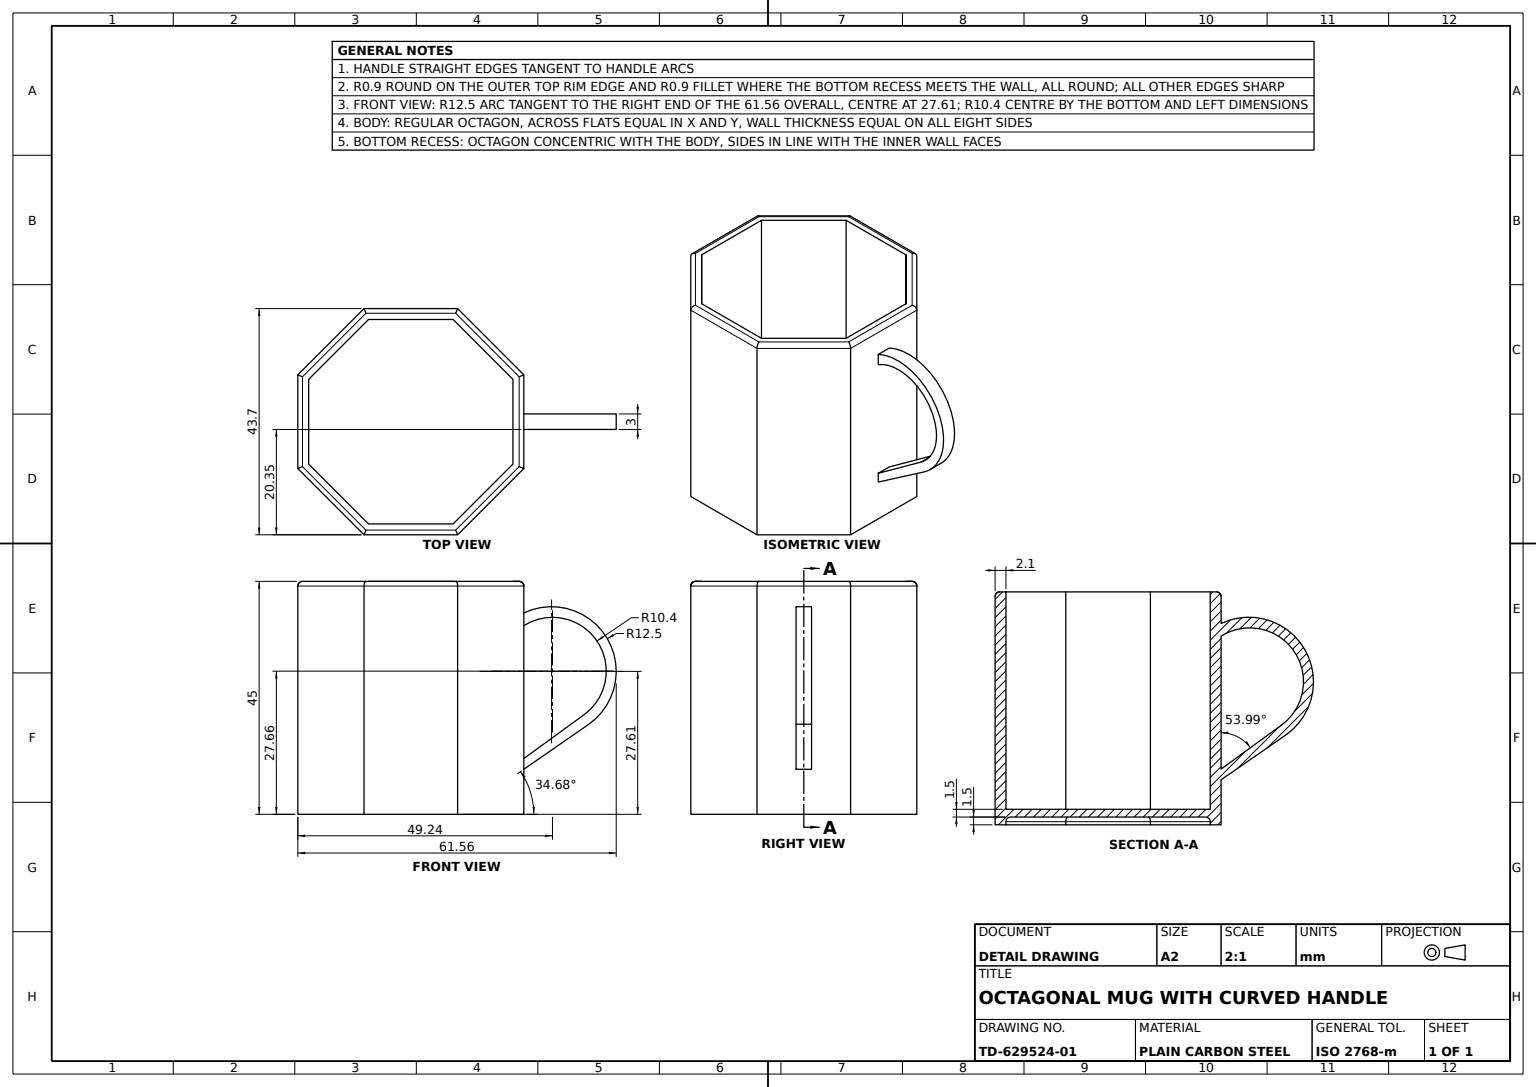
ISO-10303-21;
HEADER;
FILE_DESCRIPTION((''),'2;1');
FILE_NAME('','',(''),(''),'','','');
FILE_SCHEMA(('AUTOMOTIVE_DESIGN'));
ENDSEC;
DATA;
#1=APPLICATION_CONTEXT('');
#2=PRODUCT_CONTEXT('',#1,'mechanical');
#3=PRODUCT('','','',(#2));
#4=PRODUCT_DEFINITION_FORMATION('','',#3);
#5=PRODUCT_DEFINITION_CONTEXT('',#1,'design');
#6=PRODUCT_DEFINITION('','',#4,#5);
#7=PRODUCT_DEFINITION_SHAPE('','',#6);
#8=(LENGTH_UNIT()NAMED_UNIT(*)SI_UNIT(.MILLI.,.METRE.));
#9=(NAMED_UNIT(*)PLANE_ANGLE_UNIT()SI_UNIT($,.RADIAN.));
#10=(NAMED_UNIT(*)SI_UNIT($,.STERADIAN.)SOLID_ANGLE_UNIT());
#11=UNCERTAINTY_MEASURE_WITH_UNIT(LENGTH_MEASURE(1.E-05),#8,'distance_accuracy_value','');
#12=(GEOMETRIC_REPRESENTATION_CONTEXT(3)GLOBAL_UNCERTAINTY_ASSIGNED_CONTEXT((#11))GLOBAL_UNIT_ASSIGNED_CONTEXT((#8,#9,#10))REPRESENTATION_CONTEXT('',''));
#13=CARTESIAN_POINT('',(21.848633,44.1,9.05));
#14=VERTEX_POINT('',#13);
#15=CARTESIAN_POINT('',(9.05,44.1,21.848633));
#16=VERTEX_POINT('',#15);
#17=DIRECTION('',(-0.707106781,0.,0.707106781));
#18=VECTOR('',#17,1000.);
#19=LINE('',#15,#18);
#20=EDGE_CURVE('',#14,#16,#19,.T.);
#21=ORIENTED_EDGE('',*,*,#20,.T.);
#22=CARTESIAN_POINT('',(9.05,0.,21.848633));
#23=VERTEX_POINT('',#22);
#24=CARTESIAN_POINT('',(9.05,45.,21.848633));
#25=DIRECTION('',(0.,-1.,0.));
#26=VECTOR('',#25,1000.);
#27=LINE('',#24,#26);
#28=EDGE_CURVE('',#16,#23,#27,.T.);
#29=ORIENTED_EDGE('',*,*,#28,.T.);
#30=CARTESIAN_POINT('',(21.848633,0.,9.05));
#31=VERTEX_POINT('',#30);
#32=DIRECTION('',(0.707106781,0.,-0.707106781));
#33=VECTOR('',#32,1000.);
#34=LINE('',#22,#33);
#35=EDGE_CURVE('',#23,#31,#34,.T.);
#36=ORIENTED_EDGE('',*,*,#35,.T.);
#37=CARTESIAN_POINT('',(21.848633,45.,9.05));
#38=LINE('',#37,#26);
#39=EDGE_CURVE('',#14,#31,#38,.T.);
#40=ORIENTED_EDGE('',*,*,#39,.F.);
#41=EDGE_LOOP('',(#21,#29,#36,#40));
#42=FACE_OUTER_BOUND('',#41,.T.);
#43=DIRECTION('',(-0.707106781,0.,-0.707106781));
#44=AXIS2_PLACEMENT_3D('',#24,#43,#17);
#45=PLANE('',#44);
#46=ADVANCED_FACE('',(#42),#45,.F.);
#47=CARTESIAN_POINT('',(-9.05,44.1,21.848633));
#48=VERTEX_POINT('',#47);
#49=CARTESIAN_POINT('',(-21.848633,44.1,9.05));
#50=VERTEX_POINT('',#49);
#51=VECTOR('',#43,1000.);
#52=LINE('',#49,#51);
#53=EDGE_CURVE('',#48,#50,#52,.T.);
#54=ORIENTED_EDGE('',*,*,#53,.F.);
#55=CARTESIAN_POINT('',(-8.677208,45.,20.948633));
#56=VERTEX_POINT('',#55);
#57=CARTESIAN_POINT('',(-8.895584,45.,21.475841));
#58=CARTESIAN_POINT('',(-9.05,44.627208,21.848633));
#59=(BOUNDED_CURVE()B_SPLINE_CURVE(3,(#55,#57,#58,#47),.UNSPECIFIED.,.F.,.F.)B_SPLINE_CURVE_WITH_KNOTS((4,4),(1.570796327,3.141592654),.UNSPECIFIED.)CURVE()GEOMETRIC_REPRESENTATION_ITEM()RATIONAL_B_SPLINE_CURVE((1.,0.804737854,0.804737854,1.))REPRESENTATION_ITEM(''));
#60=EDGE_CURVE('',#56,#48,#59,.T.);
#61=ORIENTED_EDGE('',*,*,#60,.F.);
#62=CARTESIAN_POINT('',(-20.948633,45.,8.677208));
#63=VERTEX_POINT('',#62);
#64=CARTESIAN_POINT('',(-8.413604,45.,21.212237));
#65=DIRECTION('',(0.707106781,0.,0.707106781));
#66=VECTOR('',#65,1000.);
#67=LINE('',#64,#66);
#68=EDGE_CURVE('',#63,#56,#67,.T.);
#69=ORIENTED_EDGE('',*,*,#68,.F.);
#70=CARTESIAN_POINT('',(-21.475841,45.,8.895584));
#71=CARTESIAN_POINT('',(-21.848633,44.627208,9.05));
#72=(BOUNDED_CURVE()B_SPLINE_CURVE(3,(#62,#70,#71,#49),.UNSPECIFIED.,.F.,.F.)B_SPLINE_CURVE_WITH_KNOTS((4,4),(1.570796327,3.141592654),.UNSPECIFIED.)CURVE()GEOMETRIC_REPRESENTATION_ITEM()RATIONAL_B_SPLINE_CURVE((1.,0.804737854,0.804737854,1.))REPRESENTATION_ITEM(''));
#73=EDGE_CURVE('',#63,#50,#72,.T.);
#74=ORIENTED_EDGE('',*,*,#73,.T.);
#75=EDGE_LOOP('',(#54,#61,#69,#74));
#76=FACE_OUTER_BOUND('',#75,.T.);
#77=CARTESIAN_POINT('',(-14.81292,44.1,14.81292));
#78=AXIS2_PLACEMENT_3D('',#77,#43,#17);
#79=CYLINDRICAL_SURFACE('',#78,0.9);
#80=ADVANCED_FACE('',(#76),#79,.T.);
#81=CARTESIAN_POINT('',(-8.180152,45.,-19.748633));
#82=VERTEX_POINT('',#81);
#83=CARTESIAN_POINT('',(-19.748633,45.,-8.180152));
#84=VERTEX_POINT('',#83);
#85=LINE('',#81,#18);
#86=EDGE_CURVE('',#82,#84,#85,.T.);
#87=ORIENTED_EDGE('',*,*,#86,.T.);
#88=CARTESIAN_POINT('',(-19.748633,3.,-8.180152));
#89=VERTEX_POINT('',#88);
#90=LINE('',#83,#26);
#91=EDGE_CURVE('',#84,#89,#90,.T.);
#92=ORIENTED_EDGE('',*,*,#91,.T.);
#93=CARTESIAN_POINT('',(-8.180152,3.,-19.748633));
#94=VERTEX_POINT('',#93);
#95=LINE('',#88,#33);
#96=EDGE_CURVE('',#89,#94,#95,.T.);
#97=ORIENTED_EDGE('',*,*,#96,.T.);
#98=LINE('',#81,#26);
#99=EDGE_CURVE('',#82,#94,#98,.T.);
#100=ORIENTED_EDGE('',*,*,#99,.F.);
#101=EDGE_LOOP('',(#87,#92,#97,#100));
#102=FACE_OUTER_BOUND('',#101,.T.);
#103=AXIS2_PLACEMENT_3D('',#81,#65,#32);
#104=PLANE('',#103);
#105=ADVANCED_FACE('',(#102),#104,.T.);
#106=CARTESIAN_POINT('',(-19.748633,3.,8.180152));
#107=VERTEX_POINT('',#106);
#108=DIRECTION('',(0.,0.,-1.));
#109=VECTOR('',#108,1000.);
#110=LINE('',#106,#109);
#111=EDGE_CURVE('',#107,#89,#110,.T.);
#112=ORIENTED_EDGE('',*,*,#111,.F.);
#113=CARTESIAN_POINT('',(-8.180152,3.,19.748633));
#114=VERTEX_POINT('',#113);
#115=LINE('',#113,#51);
#116=EDGE_CURVE('',#114,#107,#115,.T.);
#117=ORIENTED_EDGE('',*,*,#116,.F.);
#118=CARTESIAN_POINT('',(8.180152,3.,19.748633));
#119=VERTEX_POINT('',#118);
#120=DIRECTION('',(-1.,0.,0.));
#121=VECTOR('',#120,1000.);
#122=LINE('',#118,#121);
#123=EDGE_CURVE('',#119,#114,#122,.T.);
#124=ORIENTED_EDGE('',*,*,#123,.F.);
#125=CARTESIAN_POINT('',(19.748633,3.,8.180152));
#126=VERTEX_POINT('',#125);
#127=LINE('',#125,#18);
#128=EDGE_CURVE('',#126,#119,#127,.T.);
#129=ORIENTED_EDGE('',*,*,#128,.F.);
#130=CARTESIAN_POINT('',(19.748633,3.,-8.180152));
#131=VERTEX_POINT('',#130);
#132=DIRECTION('',(0.,0.,1.));
#133=VECTOR('',#132,1000.);
#134=LINE('',#130,#133);
#135=EDGE_CURVE('',#131,#126,#134,.T.);
#136=ORIENTED_EDGE('',*,*,#135,.F.);
#137=CARTESIAN_POINT('',(8.180152,3.,-19.748633));
#138=VERTEX_POINT('',#137);
#139=LINE('',#137,#66);
#140=EDGE_CURVE('',#138,#131,#139,.T.);
#141=ORIENTED_EDGE('',*,*,#140,.F.);
#142=DIRECTION('',(1.,0.,0.));
#143=VECTOR('',#142,1000.);
#144=LINE('',#93,#143);
#145=EDGE_CURVE('',#94,#138,#144,.T.);
#146=ORIENTED_EDGE('',*,*,#145,.F.);
#147=ORIENTED_EDGE('',*,*,#96,.F.);
#148=EDGE_LOOP('',(#112,#117,#124,#129,#136,#141,#146,#147));
#149=FACE_OUTER_BOUND('',#148,.T.);
#150=CARTESIAN_POINT('',(0.,3.,0.));
#151=AXIS2_PLACEMENT_3D('',#150,#25,#108);
#152=PLANE('',#151);
#153=ADVANCED_FACE('',(#149),#152,.F.);
#154=CARTESIAN_POINT('',(19.748633,0.6,8.180152));
#155=VERTEX_POINT('',#154);
#156=CARTESIAN_POINT('',(19.748633,0.,8.180152));
#157=VERTEX_POINT('',#156);
#158=CARTESIAN_POINT('',(19.748633,45.,8.180152));
#159=LINE('',#158,#26);
#160=EDGE_CURVE('',#155,#157,#159,.T.);
#161=ORIENTED_EDGE('',*,*,#160,.F.);
#162=CARTESIAN_POINT('',(19.748633,0.6,-8.180152));
#163=VERTEX_POINT('',#162);
#164=LINE('',#162,#109);
#165=EDGE_CURVE('',#155,#163,#164,.T.);
#166=ORIENTED_EDGE('',*,*,#165,.T.);
#167=CARTESIAN_POINT('',(19.748633,0.,-8.180152));
#168=VERTEX_POINT('',#167);
#169=CARTESIAN_POINT('',(19.748633,45.,-8.180152));
#170=LINE('',#169,#26);
#171=EDGE_CURVE('',#163,#168,#170,.T.);
#172=ORIENTED_EDGE('',*,*,#171,.T.);
#173=LINE('',#156,#109);
#174=EDGE_CURVE('',#157,#168,#173,.T.);
#175=ORIENTED_EDGE('',*,*,#174,.F.);
#176=EDGE_LOOP('',(#161,#166,#172,#175));
#177=FACE_OUTER_BOUND('',#176,.T.);
#178=AXIS2_PLACEMENT_3D('',#158,#120,#132);
#179=PLANE('',#178);
#180=ADVANCED_FACE('',(#177),#179,.T.);
#181=CARTESIAN_POINT('',(-19.748633,0.6,-8.180152));
#182=VERTEX_POINT('',#181);
#183=CARTESIAN_POINT('',(-19.748633,0.,-8.180152));
#184=VERTEX_POINT('',#183);
#185=EDGE_CURVE('',#182,#184,#90,.T.);
#186=ORIENTED_EDGE('',*,*,#185,.F.);
#187=CARTESIAN_POINT('',(-19.748633,0.6,8.180152));
#188=VERTEX_POINT('',#187);
#189=LINE('',#187,#133);
#190=EDGE_CURVE('',#182,#188,#189,.T.);
#191=ORIENTED_EDGE('',*,*,#190,.T.);
#192=CARTESIAN_POINT('',(-19.748633,0.,8.180152));
#193=VERTEX_POINT('',#192);
#194=CARTESIAN_POINT('',(-19.748633,45.,8.180152));
#195=LINE('',#194,#26);
#196=EDGE_CURVE('',#188,#193,#195,.T.);
#197=ORIENTED_EDGE('',*,*,#196,.T.);
#198=LINE('',#183,#133);
#199=EDGE_CURVE('',#184,#193,#198,.T.);
#200=ORIENTED_EDGE('',*,*,#199,.F.);
#201=EDGE_LOOP('',(#186,#191,#197,#200));
#202=FACE_OUTER_BOUND('',#201,.T.);
#203=AXIS2_PLACEMENT_3D('',#83,#142,#108);
#204=PLANE('',#203);
#205=ADVANCED_FACE('',(#202),#204,.T.);
#206=CARTESIAN_POINT('',(-8.180152,45.,19.748633));
#207=VERTEX_POINT('',#206);
#208=LINE('',#206,#26);
#209=EDGE_CURVE('',#207,#114,#208,.T.);
#210=ORIENTED_EDGE('',*,*,#209,.F.);
#211=CARTESIAN_POINT('',(8.180152,45.,19.748633));
#212=VERTEX_POINT('',#211);
#213=LINE('',#206,#143);
#214=EDGE_CURVE('',#207,#212,#213,.T.);
#215=ORIENTED_EDGE('',*,*,#214,.T.);
#216=LINE('',#211,#26);
#217=EDGE_CURVE('',#212,#119,#216,.T.);
#218=ORIENTED_EDGE('',*,*,#217,.T.);
#219=ORIENTED_EDGE('',*,*,#123,.T.);
#220=EDGE_LOOP('',(#210,#215,#218,#219));
#221=FACE_OUTER_BOUND('',#220,.T.);
#222=AXIS2_PLACEMENT_3D('',#206,#108,#120);
#223=PLANE('',#222);
#224=ADVANCED_FACE('',(#221),#223,.T.);
#225=CARTESIAN_POINT('',(-21.848633,0.,-9.05));
#226=VERTEX_POINT('',#225);
#227=CARTESIAN_POINT('',(-21.848633,0.,9.05));
#228=VERTEX_POINT('',#227);
#229=LINE('',#225,#133);
#230=EDGE_CURVE('',#226,#228,#229,.T.);
#231=ORIENTED_EDGE('',*,*,#230,.T.);
#232=CARTESIAN_POINT('',(-21.848633,45.,9.05));
#233=LINE('',#232,#26);
#234=EDGE_CURVE('',#50,#228,#233,.T.);
#235=ORIENTED_EDGE('',*,*,#234,.F.);
#236=CARTESIAN_POINT('',(-21.848633,44.1,-9.05));
#237=VERTEX_POINT('',#236);
#238=LINE('',#236,#109);
#239=EDGE_CURVE('',#50,#237,#238,.T.);
#240=ORIENTED_EDGE('',*,*,#239,.T.);
#241=CARTESIAN_POINT('',(-21.848633,45.,-9.05));
#242=LINE('',#241,#26);
#243=EDGE_CURVE('',#237,#226,#242,.T.);
#244=ORIENTED_EDGE('',*,*,#243,.T.);
#245=EDGE_LOOP('',(#231,#235,#240,#244));
#246=FACE_OUTER_BOUND('',#245,.T.);
#247=AXIS2_PLACEMENT_3D('',#241,#142,#108);
#248=PLANE('',#247);
#249=ADVANCED_FACE('',(#246),#248,.F.);
#250=CARTESIAN_POINT('',(-9.05,44.1,-21.848633));
#251=VERTEX_POINT('',#250);
#252=CARTESIAN_POINT('',(-8.677208,45.,-20.948633));
#253=VERTEX_POINT('',#252);
#254=CARTESIAN_POINT('',(-9.05,44.627208,-21.848633));
#255=CARTESIAN_POINT('',(-8.895584,45.,-21.475841));
#256=(BOUNDED_CURVE()B_SPLINE_CURVE(3,(#250,#254,#255,#252),.UNSPECIFIED.,.F.,.F.)B_SPLINE_CURVE_WITH_KNOTS((4,4),(3.141592654,4.71238898),.UNSPECIFIED.)CURVE()GEOMETRIC_REPRESENTATION_ITEM()RATIONAL_B_SPLINE_CURVE((1.,0.804737854,0.804737854,1.))REPRESENTATION_ITEM(''));
#257=EDGE_CURVE('',#251,#253,#256,.T.);
#258=ORIENTED_EDGE('',*,*,#257,.F.);
#259=LINE('',#250,#33);
#260=EDGE_CURVE('',#237,#251,#259,.T.);
#261=ORIENTED_EDGE('',*,*,#260,.F.);
#262=CARTESIAN_POINT('',(-20.948633,45.,-8.677208));
#263=VERTEX_POINT('',#262);
#264=CARTESIAN_POINT('',(-21.475841,45.,-8.895584));
#265=CARTESIAN_POINT('',(-21.848633,44.627208,-9.05));
#266=(BOUNDED_CURVE()B_SPLINE_CURVE(3,(#262,#264,#265,#236),.UNSPECIFIED.,.F.,.F.)B_SPLINE_CURVE_WITH_KNOTS((4,4),(1.570796327,3.141592654),.UNSPECIFIED.)CURVE()GEOMETRIC_REPRESENTATION_ITEM()RATIONAL_B_SPLINE_CURVE((1.,0.804737854,0.804737854,1.))REPRESENTATION_ITEM(''));
#267=EDGE_CURVE('',#263,#237,#266,.T.);
#268=ORIENTED_EDGE('',*,*,#267,.F.);
#269=CARTESIAN_POINT('',(-21.212237,45.,-8.413604));
#270=LINE('',#269,#18);
#271=EDGE_CURVE('',#253,#263,#270,.T.);
#272=ORIENTED_EDGE('',*,*,#271,.F.);
#273=EDGE_LOOP('',(#258,#261,#268,#272));
#274=FACE_OUTER_BOUND('',#273,.T.);
#275=CARTESIAN_POINT('',(-14.81292,44.1,-14.81292));
#276=AXIS2_PLACEMENT_3D('',#275,#32,#43);
#277=CYLINDRICAL_SURFACE('',#276,0.9);
#278=ADVANCED_FACE('',(#274),#277,.T.);
#279=ORIENTED_EDGE('',*,*,#267,.T.);
#280=ORIENTED_EDGE('',*,*,#239,.F.);
#281=ORIENTED_EDGE('',*,*,#73,.F.);
#282=CARTESIAN_POINT('',(-20.948633,45.,9.05));
#283=LINE('',#282,#133);
#284=EDGE_CURVE('',#263,#63,#283,.T.);
#285=ORIENTED_EDGE('',*,*,#284,.F.);
#286=EDGE_LOOP('',(#279,#280,#281,#285));
#287=FACE_OUTER_BOUND('',#286,.T.);
#288=CARTESIAN_POINT('',(-20.948633,44.1,0.));
#289=AXIS2_PLACEMENT_3D('',#288,#108,#120);
#290=CYLINDRICAL_SURFACE('',#289,0.9);
#291=ADVANCED_FACE('',(#287),#290,.T.);
#292=CARTESIAN_POINT('',(7.807359,1.5,18.848633));
#293=VERTEX_POINT('',#292);
#294=CARTESIAN_POINT('',(8.180152,0.6,19.748633));
#295=VERTEX_POINT('',#294);
#296=CARTESIAN_POINT('',(8.025736,1.5,19.375841));
#297=CARTESIAN_POINT('',(8.180152,1.127208,19.748633));
#298=(BOUNDED_CURVE()B_SPLINE_CURVE(3,(#292,#296,#297,#294),.UNSPECIFIED.,.F.,.F.)B_SPLINE_CURVE_WITH_KNOTS((4,4),(4.71238898,6.283185307),.UNSPECIFIED.)CURVE()GEOMETRIC_REPRESENTATION_ITEM()RATIONAL_B_SPLINE_CURVE((1.,0.804737854,0.804737854,1.))REPRESENTATION_ITEM(''));
#299=EDGE_CURVE('',#293,#295,#298,.T.);
#300=ORIENTED_EDGE('',*,*,#299,.F.);
#301=CARTESIAN_POINT('',(18.848633,1.5,7.807359));
#302=VERTEX_POINT('',#301);
#303=CARTESIAN_POINT('',(7.543755,1.5,19.112237));
#304=LINE('',#303,#18);
#305=EDGE_CURVE('',#302,#293,#304,.T.);
#306=ORIENTED_EDGE('',*,*,#305,.F.);
#307=CARTESIAN_POINT('',(19.375841,1.5,8.025736));
#308=CARTESIAN_POINT('',(19.748633,1.127208,8.180152));
#309=(BOUNDED_CURVE()B_SPLINE_CURVE(3,(#301,#307,#308,#154),.UNSPECIFIED.,.F.,.F.)B_SPLINE_CURVE_WITH_KNOTS((4,4),(1.570796327,3.141592654),.UNSPECIFIED.)CURVE()GEOMETRIC_REPRESENTATION_ITEM()RATIONAL_B_SPLINE_CURVE((1.,0.804737854,0.804737854,1.))REPRESENTATION_ITEM(''));
#310=EDGE_CURVE('',#302,#155,#309,.T.);
#311=ORIENTED_EDGE('',*,*,#310,.T.);
#312=LINE('',#154,#33);
#313=EDGE_CURVE('',#295,#155,#312,.T.);
#314=ORIENTED_EDGE('',*,*,#313,.F.);
#315=EDGE_LOOP('',(#300,#306,#311,#314));
#316=FACE_OUTER_BOUND('',#315,.T.);
#317=CARTESIAN_POINT('',(13.327996,0.6,13.327996));
#318=AXIS2_PLACEMENT_3D('',#317,#32,#43);
#319=CYLINDRICAL_SURFACE('',#318,0.9);
#320=ADVANCED_FACE('',(#316),#319,.F.);
#321=CARTESIAN_POINT('',(21.848633,8.697939,-1.5));
#322=VERTEX_POINT('',#321);
#323=CARTESIAN_POINT('',(34.430505,17.403482,-1.5));
#324=VERTEX_POINT('',#323);
#325=CARTESIAN_POINT('',(3.003665,-4.341111,-1.5));
#326=DIRECTION('',(0.822344624,0.568989736,0.));
#327=VECTOR('',#326,1000.);
#328=LINE('',#325,#327);
#329=EDGE_CURVE('',#322,#324,#328,.T.);
#330=ORIENTED_EDGE('',*,*,#329,.T.);
#331=CARTESIAN_POINT('',(34.430505,17.403482,1.5));
#332=VERTEX_POINT('',#331);
#333=LINE('',#331,#109);
#334=EDGE_CURVE('',#332,#324,#333,.T.);
#335=ORIENTED_EDGE('',*,*,#334,.F.);
#336=CARTESIAN_POINT('',(21.848633,8.697939,1.5));
#337=VERTEX_POINT('',#336);
#338=CARTESIAN_POINT('',(3.003665,-4.341111,1.5));
#339=LINE('',#338,#327);
#340=EDGE_CURVE('',#337,#332,#339,.T.);
#341=ORIENTED_EDGE('',*,*,#340,.F.);
#342=LINE('',#336,#109);
#343=EDGE_CURVE('',#337,#322,#342,.T.);
#344=ORIENTED_EDGE('',*,*,#343,.T.);
#345=EDGE_LOOP('',(#330,#335,#341,#344));
#346=FACE_OUTER_BOUND('',#345,.T.);
#347=DIRECTION('',(-0.568989736,0.822344624,0.));
#348=DIRECTION('',(-0.822344624,-0.568989736,0.));
#349=AXIS2_PLACEMENT_3D('',#338,#347,#348);
#350=PLANE('',#349);
#351=ADVANCED_FACE('',(#346),#350,.F.);
#352=ORIENTED_EDGE('',*,*,#28,.F.);
#353=LINE('',#47,#121);
#354=EDGE_CURVE('',#16,#48,#353,.T.);
#355=ORIENTED_EDGE('',*,*,#354,.T.);
#356=CARTESIAN_POINT('',(-9.05,0.,21.848633));
#357=VERTEX_POINT('',#356);
#358=CARTESIAN_POINT('',(-9.05,45.,21.848633));
#359=LINE('',#358,#26);
#360=EDGE_CURVE('',#48,#357,#359,.T.);
#361=ORIENTED_EDGE('',*,*,#360,.T.);
#362=LINE('',#356,#143);
#363=EDGE_CURVE('',#357,#23,#362,.T.);
#364=ORIENTED_EDGE('',*,*,#363,.T.);
#365=EDGE_LOOP('',(#352,#355,#361,#364));
#366=FACE_OUTER_BOUND('',#365,.T.);
#367=AXIS2_PLACEMENT_3D('',#358,#108,#120);
#368=PLANE('',#367);
#369=ADVANCED_FACE('',(#366),#368,.F.);
#370=ORIENTED_EDGE('',*,*,#209,.T.);
#371=ORIENTED_EDGE('',*,*,#116,.T.);
#372=VERTEX_POINT('',#194);
#373=EDGE_CURVE('',#372,#107,#195,.T.);
#374=ORIENTED_EDGE('',*,*,#373,.F.);
#375=LINE('',#194,#66);
#376=EDGE_CURVE('',#372,#207,#375,.T.);
#377=ORIENTED_EDGE('',*,*,#376,.T.);
#378=EDGE_LOOP('',(#370,#371,#374,#377));
#379=FACE_OUTER_BOUND('',#378,.T.);
#380=AXIS2_PLACEMENT_3D('',#194,#32,#43);
#381=PLANE('',#380);
#382=ADVANCED_FACE('',(#379),#381,.T.);
#383=CARTESIAN_POINT('',(-8.180152,0.6,19.748633));
#384=VERTEX_POINT('',#383);
#385=CARTESIAN_POINT('',(-8.180152,0.,19.748633));
#386=VERTEX_POINT('',#385);
#387=EDGE_CURVE('',#384,#386,#208,.T.);
#388=ORIENTED_EDGE('',*,*,#387,.F.);
#389=LINE('',#294,#143);
#390=EDGE_CURVE('',#384,#295,#389,.T.);
#391=ORIENTED_EDGE('',*,*,#390,.T.);
#392=CARTESIAN_POINT('',(8.180152,0.,19.748633));
#393=VERTEX_POINT('',#392);
#394=EDGE_CURVE('',#295,#393,#216,.T.);
#395=ORIENTED_EDGE('',*,*,#394,.T.);
#396=LINE('',#385,#143);
#397=EDGE_CURVE('',#386,#393,#396,.T.);
#398=ORIENTED_EDGE('',*,*,#397,.F.);
#399=EDGE_LOOP('',(#388,#391,#395,#398));
#400=FACE_OUTER_BOUND('',#399,.T.);
#401=ADVANCED_FACE('',(#400),#223,.T.);
#402=CARTESIAN_POINT('',(8.180152,0.6,-19.748633));
#403=VERTEX_POINT('',#402);
#404=LINE('',#402,#51);
#405=EDGE_CURVE('',#163,#403,#404,.T.);
#406=ORIENTED_EDGE('',*,*,#405,.T.);
#407=CARTESIAN_POINT('',(8.180152,0.,-19.748633));
#408=VERTEX_POINT('',#407);
#409=CARTESIAN_POINT('',(8.180152,45.,-19.748633));
#410=LINE('',#409,#26);
#411=EDGE_CURVE('',#403,#408,#410,.T.);
#412=ORIENTED_EDGE('',*,*,#411,.T.);
#413=LINE('',#167,#51);
#414=EDGE_CURVE('',#168,#408,#413,.T.);
#415=ORIENTED_EDGE('',*,*,#414,.F.);
#416=ORIENTED_EDGE('',*,*,#171,.F.);
#417=EDGE_LOOP('',(#406,#412,#415,#416));
#418=FACE_OUTER_BOUND('',#417,.T.);
#419=AXIS2_PLACEMENT_3D('',#169,#17,#65);
#420=PLANE('',#419);
#421=ADVANCED_FACE('',(#418),#420,.T.);
#422=ORIENTED_EDGE('',*,*,#234,.T.);
#423=LINE('',#227,#66);
#424=EDGE_CURVE('',#228,#357,#423,.T.);
#425=ORIENTED_EDGE('',*,*,#424,.T.);
#426=ORIENTED_EDGE('',*,*,#360,.F.);
#427=ORIENTED_EDGE('',*,*,#53,.T.);
#428=EDGE_LOOP('',(#422,#425,#426,#427));
#429=FACE_OUTER_BOUND('',#428,.T.);
#430=AXIS2_PLACEMENT_3D('',#232,#32,#43);
#431=PLANE('',#430);
#432=ADVANCED_FACE('',(#429),#431,.F.);
#433=ORIENTED_EDGE('',*,*,#313,.T.);
#434=ORIENTED_EDGE('',*,*,#160,.T.);
#435=LINE('',#392,#33);
#436=EDGE_CURVE('',#393,#157,#435,.T.);
#437=ORIENTED_EDGE('',*,*,#436,.F.);
#438=ORIENTED_EDGE('',*,*,#394,.F.);
#439=EDGE_LOOP('',(#433,#434,#437,#438));
#440=FACE_OUTER_BOUND('',#439,.T.);
#441=AXIS2_PLACEMENT_3D('',#211,#43,#17);
#442=PLANE('',#441);
#443=ADVANCED_FACE('',(#440),#442,.T.);
#444=CARTESIAN_POINT('',(18.848633,1.5,-7.807359));
#445=VERTEX_POINT('',#444);
#446=CARTESIAN_POINT('',(18.848633,1.5,8.180152));
#447=LINE('',#446,#133);
#448=EDGE_CURVE('',#445,#302,#447,.T.);
#449=ORIENTED_EDGE('',*,*,#448,.T.);
#450=ORIENTED_EDGE('',*,*,#305,.T.);
#451=CARTESIAN_POINT('',(-7.807359,1.5,18.848633));
#452=VERTEX_POINT('',#451);
#453=CARTESIAN_POINT('',(-8.180152,1.5,18.848633));
#454=LINE('',#453,#121);
#455=EDGE_CURVE('',#293,#452,#454,.T.);
#456=ORIENTED_EDGE('',*,*,#455,.T.);
#457=CARTESIAN_POINT('',(-18.848633,1.5,7.807359));
#458=VERTEX_POINT('',#457);
#459=CARTESIAN_POINT('',(-19.112237,1.5,7.543755));
#460=LINE('',#459,#51);
#461=EDGE_CURVE('',#452,#458,#460,.T.);
#462=ORIENTED_EDGE('',*,*,#461,.T.);
#463=CARTESIAN_POINT('',(-18.848633,1.5,-7.807359));
#464=VERTEX_POINT('',#463);
#465=CARTESIAN_POINT('',(-18.848633,1.5,-8.180152));
#466=LINE('',#465,#109);
#467=EDGE_CURVE('',#458,#464,#466,.T.);
#468=ORIENTED_EDGE('',*,*,#467,.T.);
#469=CARTESIAN_POINT('',(-7.807359,1.5,-18.848633));
#470=VERTEX_POINT('',#469);
#471=CARTESIAN_POINT('',(-7.543755,1.5,-19.112237));
#472=LINE('',#471,#33);
#473=EDGE_CURVE('',#464,#470,#472,.T.);
#474=ORIENTED_EDGE('',*,*,#473,.T.);
#475=CARTESIAN_POINT('',(7.807359,1.5,-18.848633));
#476=VERTEX_POINT('',#475);
#477=CARTESIAN_POINT('',(8.180152,1.5,-18.848633));
#478=LINE('',#477,#143);
#479=EDGE_CURVE('',#470,#476,#478,.T.);
#480=ORIENTED_EDGE('',*,*,#479,.T.);
#481=CARTESIAN_POINT('',(19.112237,1.5,-7.543755));
#482=LINE('',#481,#66);
#483=EDGE_CURVE('',#476,#445,#482,.T.);
#484=ORIENTED_EDGE('',*,*,#483,.T.);
#485=EDGE_LOOP('',(#449,#450,#456,#462,#468,#474,#480,#484));
#486=FACE_OUTER_BOUND('',#485,.T.);
#487=CARTESIAN_POINT('',(0.,1.5,0.));
#488=AXIS2_PLACEMENT_3D('',#487,#25,#108);
#489=PLANE('',#488);
#490=ADVANCED_FACE('',(#486),#489,.T.);
#491=CARTESIAN_POINT('',(21.848633,38.90022,-1.5));
#492=VERTEX_POINT('',#491);
#493=CARTESIAN_POINT('',(27.215394,27.610939,-1.5));
#494=AXIS2_PLACEMENT_3D('',#493,#132,#142);
#495=CIRCLE('',#494,12.5);
#496=EDGE_CURVE('',#324,#492,#495,.T.);
#497=ORIENTED_EDGE('',*,*,#496,.F.);
#498=ORIENTED_EDGE('',*,*,#329,.F.);
#499=CARTESIAN_POINT('',(21.848633,10.771816,-1.5));
#500=VERTEX_POINT('',#499);
#501=CARTESIAN_POINT('',(21.848633,0.,-1.5));
#502=LINE('',#501,#26);
#503=EDGE_CURVE('',#500,#322,#502,.T.);
#504=ORIENTED_EDGE('',*,*,#503,.F.);
#505=CARTESIAN_POINT('',(33.504255,19.243632,-1.5));
#506=VERTEX_POINT('',#505);
#507=CARTESIAN_POINT('',(2.429654,-3.342746,-1.5));
#508=DIRECTION('',(-0.808901128,-0.587944695,0.));
#509=VECTOR('',#508,1000.);
#510=LINE('',#507,#509);
#511=EDGE_CURVE('',#506,#500,#510,.T.);
#512=ORIENTED_EDGE('',*,*,#511,.F.);
#513=CARTESIAN_POINT('',(21.848633,36.457189,-1.5));
#514=VERTEX_POINT('',#513);
#515=CARTESIAN_POINT('',(27.389631,27.656204,-1.5));
#516=AXIS2_PLACEMENT_3D('',#515,#132,#142);
#517=CIRCLE('',#516,10.4);
#518=EDGE_CURVE('',#506,#514,#517,.T.);
#519=ORIENTED_EDGE('',*,*,#518,.T.);
#520=EDGE_CURVE('',#492,#514,#502,.T.);
#521=ORIENTED_EDGE('',*,*,#520,.F.);
#522=EDGE_LOOP('',(#497,#498,#504,#512,#519,#521));
#523=FACE_OUTER_BOUND('',#522,.T.);
#524=CARTESIAN_POINT('',(0.,0.,-1.5));
#525=AXIS2_PLACEMENT_3D('',#524,#132,#142);
#526=PLANE('',#525);
#527=ADVANCED_FACE('',(#523),#526,.F.);
#528=ORIENTED_EDGE('',*,*,#467,.F.);
#529=CARTESIAN_POINT('',(-19.748633,1.127208,8.180152));
#530=CARTESIAN_POINT('',(-19.375841,1.5,8.025736));
#531=(BOUNDED_CURVE()B_SPLINE_CURVE(3,(#187,#529,#530,#457),.UNSPECIFIED.,.F.,.F.)B_SPLINE_CURVE_WITH_KNOTS((4,4),(3.141592654,4.71238898),.UNSPECIFIED.)CURVE()GEOMETRIC_REPRESENTATION_ITEM()RATIONAL_B_SPLINE_CURVE((1.,0.804737854,0.804737854,1.))REPRESENTATION_ITEM(''));
#532=EDGE_CURVE('',#188,#458,#531,.T.);
#533=ORIENTED_EDGE('',*,*,#532,.F.);
#534=ORIENTED_EDGE('',*,*,#190,.F.);
#535=CARTESIAN_POINT('',(-19.748633,1.127208,-8.180152));
#536=CARTESIAN_POINT('',(-19.375841,1.5,-8.025736));
#537=(BOUNDED_CURVE()B_SPLINE_CURVE(3,(#181,#535,#536,#463),.UNSPECIFIED.,.F.,.F.)B_SPLINE_CURVE_WITH_KNOTS((4,4),(3.141592654,4.71238898),.UNSPECIFIED.)CURVE()GEOMETRIC_REPRESENTATION_ITEM()RATIONAL_B_SPLINE_CURVE((1.,0.804737854,0.804737854,1.))REPRESENTATION_ITEM(''));
#538=EDGE_CURVE('',#182,#464,#537,.T.);
#539=ORIENTED_EDGE('',*,*,#538,.T.);
#540=EDGE_LOOP('',(#528,#533,#534,#539));
#541=FACE_OUTER_BOUND('',#540,.T.);
#542=CARTESIAN_POINT('',(-18.848633,0.6,0.));
#543=AXIS2_PLACEMENT_3D('',#542,#132,#142);
#544=CYLINDRICAL_SURFACE('',#543,0.9);
#545=ADVANCED_FACE('',(#541),#544,.F.);
#546=ORIENTED_EDGE('',*,*,#260,.T.);
#547=CARTESIAN_POINT('',(-9.05,0.,-21.848633));
#548=VERTEX_POINT('',#547);
#549=CARTESIAN_POINT('',(-9.05,45.,-21.848633));
#550=LINE('',#549,#26);
#551=EDGE_CURVE('',#251,#548,#550,.T.);
#552=ORIENTED_EDGE('',*,*,#551,.T.);
#553=LINE('',#547,#18);
#554=EDGE_CURVE('',#548,#226,#553,.T.);
#555=ORIENTED_EDGE('',*,*,#554,.T.);
#556=ORIENTED_EDGE('',*,*,#243,.F.);
#557=EDGE_LOOP('',(#546,#552,#555,#556));
#558=FACE_OUTER_BOUND('',#557,.T.);
#559=AXIS2_PLACEMENT_3D('',#549,#65,#32);
#560=PLANE('',#559);
#561=ADVANCED_FACE('',(#558),#560,.F.);
#562=CARTESIAN_POINT('',(20.948633,45.,8.677208));
#563=VERTEX_POINT('',#562);
#564=CARTESIAN_POINT('',(21.848633,44.627208,9.05));
#565=CARTESIAN_POINT('',(21.475841,45.,8.895584));
#566=(BOUNDED_CURVE()B_SPLINE_CURVE(3,(#13,#564,#565,#562),.UNSPECIFIED.,.F.,.F.)B_SPLINE_CURVE_WITH_KNOTS((4,4),(0.,1.570796327),.UNSPECIFIED.)CURVE()GEOMETRIC_REPRESENTATION_ITEM()RATIONAL_B_SPLINE_CURVE((1.,0.804737854,0.804737854,1.))REPRESENTATION_ITEM(''));
#567=EDGE_CURVE('',#14,#563,#566,.T.);
#568=ORIENTED_EDGE('',*,*,#567,.T.);
#569=CARTESIAN_POINT('',(8.677208,45.,20.948633));
#570=VERTEX_POINT('',#569);
#571=CARTESIAN_POINT('',(21.212237,45.,8.413604));
#572=LINE('',#571,#33);
#573=EDGE_CURVE('',#570,#563,#572,.T.);
#574=ORIENTED_EDGE('',*,*,#573,.F.);
#575=CARTESIAN_POINT('',(8.895584,45.,21.475841));
#576=CARTESIAN_POINT('',(9.05,44.627208,21.848633));
#577=(BOUNDED_CURVE()B_SPLINE_CURVE(3,(#569,#575,#576,#15),.UNSPECIFIED.,.F.,.F.)B_SPLINE_CURVE_WITH_KNOTS((4,4),(1.570796327,3.141592654),.UNSPECIFIED.)CURVE()GEOMETRIC_REPRESENTATION_ITEM()RATIONAL_B_SPLINE_CURVE((1.,0.804737854,0.804737854,1.))REPRESENTATION_ITEM(''));
#578=EDGE_CURVE('',#570,#16,#577,.T.);
#579=ORIENTED_EDGE('',*,*,#578,.T.);
#580=ORIENTED_EDGE('',*,*,#20,.F.);
#581=EDGE_LOOP('',(#568,#574,#579,#580));
#582=FACE_OUTER_BOUND('',#581,.T.);
#583=CARTESIAN_POINT('',(14.81292,44.1,14.81292));
#584=AXIS2_PLACEMENT_3D('',#583,#17,#65);
#585=CYLINDRICAL_SURFACE('',#584,0.9);
#586=ADVANCED_FACE('',(#582),#585,.T.);
#587=ORIENTED_EDGE('',*,*,#99,.T.);
#588=ORIENTED_EDGE('',*,*,#145,.T.);
#589=VERTEX_POINT('',#409);
#590=EDGE_CURVE('',#589,#138,#410,.T.);
#591=ORIENTED_EDGE('',*,*,#590,.F.);
#592=LINE('',#409,#121);
#593=EDGE_CURVE('',#589,#82,#592,.T.);
#594=ORIENTED_EDGE('',*,*,#593,.T.);
#595=EDGE_LOOP('',(#587,#588,#591,#594));
#596=FACE_OUTER_BOUND('',#595,.T.);
#597=AXIS2_PLACEMENT_3D('',#409,#132,#142);
#598=PLANE('',#597);
#599=ADVANCED_FACE('',(#596),#598,.T.);
#600=ORIENTED_EDGE('',*,*,#578,.F.);
#601=CARTESIAN_POINT('',(9.05,45.,20.948633));
#602=LINE('',#601,#143);
#603=EDGE_CURVE('',#56,#570,#602,.T.);
#604=ORIENTED_EDGE('',*,*,#603,.F.);
#605=ORIENTED_EDGE('',*,*,#60,.T.);
#606=ORIENTED_EDGE('',*,*,#354,.F.);
#607=EDGE_LOOP('',(#600,#604,#605,#606));
#608=FACE_OUTER_BOUND('',#607,.T.);
#609=CARTESIAN_POINT('',(0.,44.1,20.948633));
#610=AXIS2_PLACEMENT_3D('',#609,#120,#132);
#611=CYLINDRICAL_SURFACE('',#610,0.9);
#612=ADVANCED_FACE('',(#608),#611,.T.);
#613=ORIENTED_EDGE('',*,*,#373,.T.);
#614=ORIENTED_EDGE('',*,*,#111,.T.);
#615=ORIENTED_EDGE('',*,*,#91,.F.);
#616=LINE('',#83,#133);
#617=EDGE_CURVE('',#84,#372,#616,.T.);
#618=ORIENTED_EDGE('',*,*,#617,.T.);
#619=EDGE_LOOP('',(#613,#614,#615,#618));
#620=FACE_OUTER_BOUND('',#619,.T.);
#621=ADVANCED_FACE('',(#620),#204,.T.);
#622=CARTESIAN_POINT('',(21.848633,38.90022,1.5));
#623=VERTEX_POINT('',#622);
#624=CARTESIAN_POINT('',(27.215394,27.610939,1.5));
#625=AXIS2_PLACEMENT_3D('',#624,#132,#142);
#626=CIRCLE('',#625,12.5);
#627=EDGE_CURVE('',#332,#623,#626,.T.);
#628=ORIENTED_EDGE('',*,*,#627,.T.);
#629=CARTESIAN_POINT('',(21.848633,36.457189,1.5));
#630=VERTEX_POINT('',#629);
#631=CARTESIAN_POINT('',(21.848633,0.,1.5));
#632=LINE('',#631,#26);
#633=EDGE_CURVE('',#623,#630,#632,.T.);
#634=ORIENTED_EDGE('',*,*,#633,.T.);
#635=CARTESIAN_POINT('',(33.504255,19.243632,1.5));
#636=VERTEX_POINT('',#635);
#637=CARTESIAN_POINT('',(27.389631,27.656204,1.5));
#638=AXIS2_PLACEMENT_3D('',#637,#132,#142);
#639=CIRCLE('',#638,10.4);
#640=EDGE_CURVE('',#636,#630,#639,.T.);
#641=ORIENTED_EDGE('',*,*,#640,.F.);
#642=CARTESIAN_POINT('',(21.848633,10.771816,1.5));
#643=VERTEX_POINT('',#642);
#644=CARTESIAN_POINT('',(2.429654,-3.342746,1.5));
#645=LINE('',#644,#509);
#646=EDGE_CURVE('',#636,#643,#645,.T.);
#647=ORIENTED_EDGE('',*,*,#646,.T.);
#648=EDGE_CURVE('',#643,#337,#632,.T.);
#649=ORIENTED_EDGE('',*,*,#648,.T.);
#650=ORIENTED_EDGE('',*,*,#340,.T.);
#651=EDGE_LOOP('',(#628,#634,#641,#647,#649,#650));
#652=FACE_OUTER_BOUND('',#651,.T.);
#653=CARTESIAN_POINT('',(0.,0.,1.5));
#654=AXIS2_PLACEMENT_3D('',#653,#132,#142);
#655=PLANE('',#654);
#656=ADVANCED_FACE('',(#652),#655,.T.);
#657=ORIENTED_EDGE('',*,*,#174,.T.);
#658=ORIENTED_EDGE('',*,*,#414,.T.);
#659=CARTESIAN_POINT('',(-8.180152,0.,-19.748633));
#660=VERTEX_POINT('',#659);
#661=LINE('',#407,#121);
#662=EDGE_CURVE('',#408,#660,#661,.T.);
#663=ORIENTED_EDGE('',*,*,#662,.T.);
#664=LINE('',#659,#18);
#665=EDGE_CURVE('',#660,#184,#664,.T.);
#666=ORIENTED_EDGE('',*,*,#665,.T.);
#667=ORIENTED_EDGE('',*,*,#199,.T.);
#668=LINE('',#192,#66);
#669=EDGE_CURVE('',#193,#386,#668,.T.);
#670=ORIENTED_EDGE('',*,*,#669,.T.);
#671=ORIENTED_EDGE('',*,*,#397,.T.);
#672=ORIENTED_EDGE('',*,*,#436,.T.);
#673=EDGE_LOOP('',(#657,#658,#663,#666,#667,#670,#671,#672));
#674=FACE_BOUND('',#673,.T.);
#675=ORIENTED_EDGE('',*,*,#230,.F.);
#676=ORIENTED_EDGE('',*,*,#554,.F.);
#677=CARTESIAN_POINT('',(9.05,0.,-21.848633));
#678=VERTEX_POINT('',#677);
#679=LINE('',#677,#121);
#680=EDGE_CURVE('',#678,#548,#679,.T.);
#681=ORIENTED_EDGE('',*,*,#680,.F.);
#682=CARTESIAN_POINT('',(21.848633,0.,-9.05));
#683=VERTEX_POINT('',#682);
#684=LINE('',#682,#51);
#685=EDGE_CURVE('',#683,#678,#684,.T.);
#686=ORIENTED_EDGE('',*,*,#685,.F.);
#687=LINE('',#30,#109);
#688=EDGE_CURVE('',#31,#683,#687,.T.);
#689=ORIENTED_EDGE('',*,*,#688,.F.);
#690=ORIENTED_EDGE('',*,*,#35,.F.);
#691=ORIENTED_EDGE('',*,*,#363,.F.);
#692=ORIENTED_EDGE('',*,*,#424,.F.);
#693=EDGE_LOOP('',(#675,#676,#681,#686,#689,#690,#691,#692));
#694=FACE_OUTER_BOUND('',#693,.T.);
#695=CARTESIAN_POINT('',(0.,0.,0.));
#696=DIRECTION('',(0.,1.,0.));
#697=AXIS2_PLACEMENT_3D('',#695,#696,#132);
#698=PLANE('',#697);
#699=ADVANCED_FACE('',(#674,#694),#698,.F.);
#700=ORIENTED_EDGE('',*,*,#140,.T.);
#701=VERTEX_POINT('',#169);
#702=EDGE_CURVE('',#701,#131,#170,.T.);
#703=ORIENTED_EDGE('',*,*,#702,.F.);
#704=LINE('',#169,#51);
#705=EDGE_CURVE('',#701,#589,#704,.T.);
#706=ORIENTED_EDGE('',*,*,#705,.T.);
#707=ORIENTED_EDGE('',*,*,#590,.T.);
#708=EDGE_LOOP('',(#700,#703,#706,#707));
#709=FACE_OUTER_BOUND('',#708,.T.);
#710=ADVANCED_FACE('',(#709),#420,.T.);
#711=ORIENTED_EDGE('',*,*,#185,.T.);
#712=ORIENTED_EDGE('',*,*,#665,.F.);
#713=CARTESIAN_POINT('',(-8.180152,0.6,-19.748633));
#714=VERTEX_POINT('',#713);
#715=EDGE_CURVE('',#714,#660,#98,.T.);
#716=ORIENTED_EDGE('',*,*,#715,.F.);
#717=LINE('',#181,#18);
#718=EDGE_CURVE('',#714,#182,#717,.T.);
#719=ORIENTED_EDGE('',*,*,#718,.T.);
#720=EDGE_LOOP('',(#711,#712,#716,#719));
#721=FACE_OUTER_BOUND('',#720,.T.);
#722=ADVANCED_FACE('',(#721),#104,.T.);
#723=ORIENTED_EDGE('',*,*,#669,.F.);
#724=ORIENTED_EDGE('',*,*,#196,.F.);
#725=LINE('',#383,#66);
#726=EDGE_CURVE('',#188,#384,#725,.T.);
#727=ORIENTED_EDGE('',*,*,#726,.T.);
#728=ORIENTED_EDGE('',*,*,#387,.T.);
#729=EDGE_LOOP('',(#723,#724,#727,#728));
#730=FACE_OUTER_BOUND('',#729,.T.);
#731=ADVANCED_FACE('',(#730),#381,.T.);
#732=LINE('',#629,#109);
#733=EDGE_CURVE('',#630,#514,#732,.T.);
#734=ORIENTED_EDGE('',*,*,#733,.F.);
#735=ORIENTED_EDGE('',*,*,#633,.F.);
#736=LINE('',#622,#109);
#737=EDGE_CURVE('',#623,#492,#736,.T.);
#738=ORIENTED_EDGE('',*,*,#737,.T.);
#739=ORIENTED_EDGE('',*,*,#520,.T.);
#740=EDGE_LOOP('',(#734,#735,#738,#739));
#741=FACE_BOUND('',#740,.T.);
#742=ORIENTED_EDGE('',*,*,#39,.T.);
#743=ORIENTED_EDGE('',*,*,#688,.T.);
#744=CARTESIAN_POINT('',(21.848633,44.1,-9.05));
#745=VERTEX_POINT('',#744);
#746=CARTESIAN_POINT('',(21.848633,45.,-9.05));
#747=LINE('',#746,#26);
#748=EDGE_CURVE('',#745,#683,#747,.T.);
#749=ORIENTED_EDGE('',*,*,#748,.F.);
#750=LINE('',#13,#133);
#751=EDGE_CURVE('',#745,#14,#750,.T.);
#752=ORIENTED_EDGE('',*,*,#751,.T.);
#753=EDGE_LOOP('',(#742,#743,#749,#752));
#754=FACE_OUTER_BOUND('',#753,.T.);
#755=ORIENTED_EDGE('',*,*,#503,.T.);
#756=ORIENTED_EDGE('',*,*,#343,.F.);
#757=ORIENTED_EDGE('',*,*,#648,.F.);
#758=LINE('',#642,#109);
#759=EDGE_CURVE('',#643,#500,#758,.T.);
#760=ORIENTED_EDGE('',*,*,#759,.T.);
#761=EDGE_LOOP('',(#755,#756,#757,#760));
#762=FACE_BOUND('',#761,.T.);
#763=AXIS2_PLACEMENT_3D('',#37,#120,#132);
#764=PLANE('',#763);
#765=ADVANCED_FACE('',(#741,#754,#762),#764,.F.);
#766=ORIENTED_EDGE('',*,*,#86,.F.);
#767=ORIENTED_EDGE('',*,*,#593,.F.);
#768=ORIENTED_EDGE('',*,*,#705,.F.);
#769=VERTEX_POINT('',#158);
#770=LINE('',#158,#109);
#771=EDGE_CURVE('',#769,#701,#770,.T.);
#772=ORIENTED_EDGE('',*,*,#771,.F.);
#773=LINE('',#211,#33);
#774=EDGE_CURVE('',#212,#769,#773,.T.);
#775=ORIENTED_EDGE('',*,*,#774,.F.);
#776=ORIENTED_EDGE('',*,*,#214,.F.);
#777=ORIENTED_EDGE('',*,*,#376,.F.);
#778=ORIENTED_EDGE('',*,*,#617,.F.);
#779=EDGE_LOOP('',(#766,#767,#768,#772,#775,#776,#777,#778));
#780=FACE_BOUND('',#779,.T.);
#781=ORIENTED_EDGE('',*,*,#284,.T.);
#782=ORIENTED_EDGE('',*,*,#68,.T.);
#783=ORIENTED_EDGE('',*,*,#603,.T.);
#784=ORIENTED_EDGE('',*,*,#573,.T.);
#785=CARTESIAN_POINT('',(20.948633,45.,-8.677208));
#786=VERTEX_POINT('',#785);
#787=CARTESIAN_POINT('',(20.948633,45.,-9.05));
#788=LINE('',#787,#109);
#789=EDGE_CURVE('',#563,#786,#788,.T.);
#790=ORIENTED_EDGE('',*,*,#789,.T.);
#791=CARTESIAN_POINT('',(8.677208,45.,-20.948633));
#792=VERTEX_POINT('',#791);
#793=CARTESIAN_POINT('',(8.413604,45.,-21.212237));
#794=LINE('',#793,#51);
#795=EDGE_CURVE('',#786,#792,#794,.T.);
#796=ORIENTED_EDGE('',*,*,#795,.T.);
#797=CARTESIAN_POINT('',(-9.05,45.,-20.948633));
#798=LINE('',#797,#121);
#799=EDGE_CURVE('',#792,#253,#798,.T.);
#800=ORIENTED_EDGE('',*,*,#799,.T.);
#801=ORIENTED_EDGE('',*,*,#271,.T.);
#802=EDGE_LOOP('',(#781,#782,#783,#784,#790,#796,#800,#801));
#803=FACE_OUTER_BOUND('',#802,.T.);
#804=CARTESIAN_POINT('',(0.,45.,0.));
#805=AXIS2_PLACEMENT_3D('',#804,#696,#132);
#806=PLANE('',#805);
#807=ADVANCED_FACE('',(#780,#803),#806,.T.);
#808=ORIENTED_EDGE('',*,*,#299,.T.);
#809=ORIENTED_EDGE('',*,*,#390,.F.);
#810=CARTESIAN_POINT('',(-8.180152,1.127208,19.748633));
#811=CARTESIAN_POINT('',(-8.025736,1.5,19.375841));
#812=(BOUNDED_CURVE()B_SPLINE_CURVE(3,(#383,#810,#811,#451),.UNSPECIFIED.,.F.,.F.)B_SPLINE_CURVE_WITH_KNOTS((4,4),(3.141592654,4.71238898),.UNSPECIFIED.)CURVE()GEOMETRIC_REPRESENTATION_ITEM()RATIONAL_B_SPLINE_CURVE((1.,0.804737854,0.804737854,1.))REPRESENTATION_ITEM(''));
#813=EDGE_CURVE('',#384,#452,#812,.T.);
#814=ORIENTED_EDGE('',*,*,#813,.T.);
#815=ORIENTED_EDGE('',*,*,#455,.F.);
#816=EDGE_LOOP('',(#808,#809,#814,#815));
#817=FACE_OUTER_BOUND('',#816,.T.);
#818=CARTESIAN_POINT('',(0.,0.6,18.848633));
#819=AXIS2_PLACEMENT_3D('',#818,#142,#108);
#820=CYLINDRICAL_SURFACE('',#819,0.9);
#821=ADVANCED_FACE('',(#817),#820,.F.);
#822=ORIENTED_EDGE('',*,*,#518,.F.);
#823=LINE('',#635,#109);
#824=EDGE_CURVE('',#636,#506,#823,.T.);
#825=ORIENTED_EDGE('',*,*,#824,.F.);
#826=ORIENTED_EDGE('',*,*,#640,.T.);
#827=ORIENTED_EDGE('',*,*,#733,.T.);
#828=EDGE_LOOP('',(#822,#825,#826,#827));
#829=FACE_OUTER_BOUND('',#828,.T.);
#830=AXIS2_PLACEMENT_3D('',#637,#108,#120);
#831=CYLINDRICAL_SURFACE('',#830,10.4);
#832=ADVANCED_FACE('',(#829),#831,.F.);
#833=ORIENTED_EDGE('',*,*,#715,.T.);
#834=ORIENTED_EDGE('',*,*,#662,.F.);
#835=ORIENTED_EDGE('',*,*,#411,.F.);
#836=LINE('',#713,#121);
#837=EDGE_CURVE('',#403,#714,#836,.T.);
#838=ORIENTED_EDGE('',*,*,#837,.T.);
#839=EDGE_LOOP('',(#833,#834,#835,#838));
#840=FACE_OUTER_BOUND('',#839,.T.);
#841=ADVANCED_FACE('',(#840),#598,.T.);
#842=ORIENTED_EDGE('',*,*,#680,.T.);
#843=ORIENTED_EDGE('',*,*,#551,.F.);
#844=CARTESIAN_POINT('',(9.05,44.1,-21.848633));
#845=VERTEX_POINT('',#844);
#846=LINE('',#844,#143);
#847=EDGE_CURVE('',#251,#845,#846,.T.);
#848=ORIENTED_EDGE('',*,*,#847,.T.);
#849=CARTESIAN_POINT('',(9.05,45.,-21.848633));
#850=LINE('',#849,#26);
#851=EDGE_CURVE('',#845,#678,#850,.T.);
#852=ORIENTED_EDGE('',*,*,#851,.T.);
#853=EDGE_LOOP('',(#842,#843,#848,#852));
#854=FACE_OUTER_BOUND('',#853,.T.);
#855=AXIS2_PLACEMENT_3D('',#849,#132,#142);
#856=PLANE('',#855);
#857=ADVANCED_FACE('',(#854),#856,.F.);
#858=ORIENTED_EDGE('',*,*,#128,.T.);
#859=ORIENTED_EDGE('',*,*,#217,.F.);
#860=ORIENTED_EDGE('',*,*,#774,.T.);
#861=EDGE_CURVE('',#769,#126,#159,.T.);
#862=ORIENTED_EDGE('',*,*,#861,.T.);
#863=EDGE_LOOP('',(#858,#859,#860,#862));
#864=FACE_OUTER_BOUND('',#863,.T.);
#865=ADVANCED_FACE('',(#864),#442,.T.);
#866=CARTESIAN_POINT('',(-8.180152,1.127208,-19.748633));
#867=CARTESIAN_POINT('',(-8.025736,1.5,-19.375841));
#868=(BOUNDED_CURVE()B_SPLINE_CURVE(3,(#713,#866,#867,#469),.UNSPECIFIED.,.F.,.T.)B_SPLINE_CURVE_WITH_KNOTS((4,4),(3.141592654,4.71238898),.UNSPECIFIED.)CURVE()GEOMETRIC_REPRESENTATION_ITEM()RATIONAL_B_SPLINE_CURVE((1.,0.804737854,0.804737854,1.))REPRESENTATION_ITEM(''));
#869=EDGE_CURVE('',#714,#470,#868,.T.);
#870=ORIENTED_EDGE('',*,*,#869,.T.);
#871=ORIENTED_EDGE('',*,*,#473,.F.);
#872=ORIENTED_EDGE('',*,*,#538,.F.);
#873=ORIENTED_EDGE('',*,*,#718,.F.);
#874=EDGE_LOOP('',(#870,#871,#872,#873));
#875=FACE_OUTER_BOUND('',#874,.T.);
#876=CARTESIAN_POINT('',(-13.327996,0.6,-13.327996));
#877=AXIS2_PLACEMENT_3D('',#876,#17,#65);
#878=CYLINDRICAL_SURFACE('',#877,0.9);
#879=ADVANCED_FACE('',(#875),#878,.F.);
#880=ORIENTED_EDGE('',*,*,#135,.T.);
#881=ORIENTED_EDGE('',*,*,#861,.F.);
#882=ORIENTED_EDGE('',*,*,#771,.T.);
#883=ORIENTED_EDGE('',*,*,#702,.T.);
#884=EDGE_LOOP('',(#880,#881,#882,#883));
#885=FACE_OUTER_BOUND('',#884,.T.);
#886=ADVANCED_FACE('',(#885),#179,.T.);
#887=ORIENTED_EDGE('',*,*,#461,.F.);
#888=ORIENTED_EDGE('',*,*,#813,.F.);
#889=ORIENTED_EDGE('',*,*,#726,.F.);
#890=ORIENTED_EDGE('',*,*,#532,.T.);
#891=EDGE_LOOP('',(#887,#888,#889,#890));
#892=FACE_OUTER_BOUND('',#891,.T.);
#893=CARTESIAN_POINT('',(-13.327996,0.6,13.327996));
#894=AXIS2_PLACEMENT_3D('',#893,#65,#32);
#895=CYLINDRICAL_SURFACE('',#894,0.9);
#896=ADVANCED_FACE('',(#892),#895,.F.);
#897=ORIENTED_EDGE('',*,*,#405,.F.);
#898=CARTESIAN_POINT('',(19.375841,1.5,-8.025736));
#899=CARTESIAN_POINT('',(19.748633,1.127208,-8.180152));
#900=(BOUNDED_CURVE()B_SPLINE_CURVE(3,(#444,#898,#899,#162),.UNSPECIFIED.,.F.,.F.)B_SPLINE_CURVE_WITH_KNOTS((4,4),(1.570796327,3.141592654),.UNSPECIFIED.)CURVE()GEOMETRIC_REPRESENTATION_ITEM()RATIONAL_B_SPLINE_CURVE((1.,0.804737854,0.804737854,1.))REPRESENTATION_ITEM(''));
#901=EDGE_CURVE('',#445,#163,#900,.T.);
#902=ORIENTED_EDGE('',*,*,#901,.F.);
#903=ORIENTED_EDGE('',*,*,#483,.F.);
#904=CARTESIAN_POINT('',(8.025736,1.5,-19.375841));
#905=CARTESIAN_POINT('',(8.180152,1.127208,-19.748633));
#906=(BOUNDED_CURVE()B_SPLINE_CURVE(3,(#475,#904,#905,#402),.UNSPECIFIED.,.F.,.F.)B_SPLINE_CURVE_WITH_KNOTS((4,4),(1.570796327,3.141592654),.UNSPECIFIED.)CURVE()GEOMETRIC_REPRESENTATION_ITEM()RATIONAL_B_SPLINE_CURVE((1.,0.804737854,0.804737854,1.))REPRESENTATION_ITEM(''));
#907=EDGE_CURVE('',#476,#403,#906,.T.);
#908=ORIENTED_EDGE('',*,*,#907,.T.);
#909=EDGE_LOOP('',(#897,#902,#903,#908));
#910=FACE_OUTER_BOUND('',#909,.T.);
#911=CARTESIAN_POINT('',(13.327996,0.6,-13.327996));
#912=AXIS2_PLACEMENT_3D('',#911,#43,#17);
#913=CYLINDRICAL_SURFACE('',#912,0.9);
#914=ADVANCED_FACE('',(#910),#913,.F.);
#915=ORIENTED_EDGE('',*,*,#685,.T.);
#916=ORIENTED_EDGE('',*,*,#851,.F.);
#917=LINE('',#744,#66);
#918=EDGE_CURVE('',#845,#745,#917,.T.);
#919=ORIENTED_EDGE('',*,*,#918,.T.);
#920=ORIENTED_EDGE('',*,*,#748,.T.);
#921=EDGE_LOOP('',(#915,#916,#919,#920));
#922=FACE_OUTER_BOUND('',#921,.T.);
#923=AXIS2_PLACEMENT_3D('',#746,#17,#65);
#924=PLANE('',#923);
#925=ADVANCED_FACE('',(#922),#924,.F.);
#926=ORIENTED_EDGE('',*,*,#165,.F.);
#927=ORIENTED_EDGE('',*,*,#310,.F.);
#928=ORIENTED_EDGE('',*,*,#448,.F.);
#929=ORIENTED_EDGE('',*,*,#901,.T.);
#930=EDGE_LOOP('',(#926,#927,#928,#929));
#931=FACE_OUTER_BOUND('',#930,.T.);
#932=CARTESIAN_POINT('',(18.848633,0.6,0.));
#933=AXIS2_PLACEMENT_3D('',#932,#108,#120);
#934=CYLINDRICAL_SURFACE('',#933,0.9);
#935=ADVANCED_FACE('',(#931),#934,.F.);
#936=ORIENTED_EDGE('',*,*,#837,.F.);
#937=ORIENTED_EDGE('',*,*,#907,.F.);
#938=ORIENTED_EDGE('',*,*,#479,.F.);
#939=ORIENTED_EDGE('',*,*,#869,.F.);
#940=EDGE_LOOP('',(#936,#937,#938,#939));
#941=FACE_OUTER_BOUND('',#940,.T.);
#942=CARTESIAN_POINT('',(0.,0.6,-18.848633));
#943=AXIS2_PLACEMENT_3D('',#942,#120,#132);
#944=CYLINDRICAL_SURFACE('',#943,0.9);
#945=ADVANCED_FACE('',(#941),#944,.F.);
#946=CARTESIAN_POINT('',(21.848633,44.627208,-9.05));
#947=CARTESIAN_POINT('',(21.475841,45.,-8.895584));
#948=(BOUNDED_CURVE()B_SPLINE_CURVE(3,(#744,#946,#947,#785),.UNSPECIFIED.,.F.,.F.)B_SPLINE_CURVE_WITH_KNOTS((4,4),(3.141592654,4.71238898),.UNSPECIFIED.)CURVE()GEOMETRIC_REPRESENTATION_ITEM()RATIONAL_B_SPLINE_CURVE((1.,0.804737854,0.804737854,1.))REPRESENTATION_ITEM(''));
#949=EDGE_CURVE('',#745,#786,#948,.T.);
#950=ORIENTED_EDGE('',*,*,#949,.F.);
#951=ORIENTED_EDGE('',*,*,#918,.F.);
#952=CARTESIAN_POINT('',(9.05,44.627208,-21.848633));
#953=CARTESIAN_POINT('',(8.895584,45.,-21.475841));
#954=(BOUNDED_CURVE()B_SPLINE_CURVE(3,(#844,#952,#953,#791),.UNSPECIFIED.,.F.,.F.)B_SPLINE_CURVE_WITH_KNOTS((4,4),(3.141592654,4.71238898),.UNSPECIFIED.)CURVE()GEOMETRIC_REPRESENTATION_ITEM()RATIONAL_B_SPLINE_CURVE((1.,0.804737854,0.804737854,1.))REPRESENTATION_ITEM(''));
#955=EDGE_CURVE('',#845,#792,#954,.T.);
#956=ORIENTED_EDGE('',*,*,#955,.T.);
#957=ORIENTED_EDGE('',*,*,#795,.F.);
#958=EDGE_LOOP('',(#950,#951,#956,#957));
#959=FACE_OUTER_BOUND('',#958,.T.);
#960=CARTESIAN_POINT('',(14.81292,44.1,-14.81292));
#961=AXIS2_PLACEMENT_3D('',#960,#65,#32);
#962=CYLINDRICAL_SURFACE('',#961,0.9);
#963=ADVANCED_FACE('',(#959),#962,.T.);
#964=ORIENTED_EDGE('',*,*,#824,.T.);
#965=ORIENTED_EDGE('',*,*,#511,.T.);
#966=ORIENTED_EDGE('',*,*,#759,.F.);
#967=ORIENTED_EDGE('',*,*,#646,.F.);
#968=EDGE_LOOP('',(#964,#965,#966,#967));
#969=FACE_OUTER_BOUND('',#968,.T.);
#970=DIRECTION('',(0.587944695,-0.808901128,0.));
#971=DIRECTION('',(0.808901128,0.587944695,0.));
#972=AXIS2_PLACEMENT_3D('',#644,#970,#971);
#973=PLANE('',#972);
#974=ADVANCED_FACE('',(#969),#973,.F.);
#975=ORIENTED_EDGE('',*,*,#567,.F.);
#976=ORIENTED_EDGE('',*,*,#751,.F.);
#977=ORIENTED_EDGE('',*,*,#949,.T.);
#978=ORIENTED_EDGE('',*,*,#789,.F.);
#979=EDGE_LOOP('',(#975,#976,#977,#978));
#980=FACE_OUTER_BOUND('',#979,.T.);
#981=CARTESIAN_POINT('',(20.948633,44.1,0.));
#982=AXIS2_PLACEMENT_3D('',#981,#132,#142);
#983=CYLINDRICAL_SURFACE('',#982,0.9);
#984=ADVANCED_FACE('',(#980),#983,.T.);
#985=ORIENTED_EDGE('',*,*,#847,.F.);
#986=ORIENTED_EDGE('',*,*,#257,.T.);
#987=ORIENTED_EDGE('',*,*,#799,.F.);
#988=ORIENTED_EDGE('',*,*,#955,.F.);
#989=EDGE_LOOP('',(#985,#986,#987,#988));
#990=FACE_OUTER_BOUND('',#989,.T.);
#991=CARTESIAN_POINT('',(0.,44.1,-20.948633));
#992=AXIS2_PLACEMENT_3D('',#991,#142,#108);
#993=CYLINDRICAL_SURFACE('',#992,0.9);
#994=ADVANCED_FACE('',(#990),#993,.T.);
#995=ORIENTED_EDGE('',*,*,#737,.F.);
#996=ORIENTED_EDGE('',*,*,#627,.F.);
#997=ORIENTED_EDGE('',*,*,#334,.T.);
#998=ORIENTED_EDGE('',*,*,#496,.T.);
#999=EDGE_LOOP('',(#995,#996,#997,#998));
#1000=FACE_OUTER_BOUND('',#999,.T.);
#1001=AXIS2_PLACEMENT_3D('',#624,#108,#120);
#1002=CYLINDRICAL_SURFACE('',#1001,12.5);
#1003=ADVANCED_FACE('',(#1000),#1002,.T.);
#1004=CLOSED_SHELL('',(#46,#80,#105,#153,#180,#205,#224,#249,#278,#291,#320,#351,#369,#382,#401,#421,#432,#443,#490,#527,#545,#561,#586,#599,#612,#621,#656,#699,#710,#722,#731,#765,#807,#821,#832,#841,#857,#865,#879,#886,#896,#914,#925,#935,#945,#963,#974,#984,#994,#1003));
#1005=MANIFOLD_SOLID_BREP('',#1004);
#1006=ADVANCED_BREP_SHAPE_REPRESENTATION('',(#1005),#12);
#1007=SHAPE_DEFINITION_REPRESENTATION(#7,#1006);
ENDSEC;
END-ISO-10303-21;
